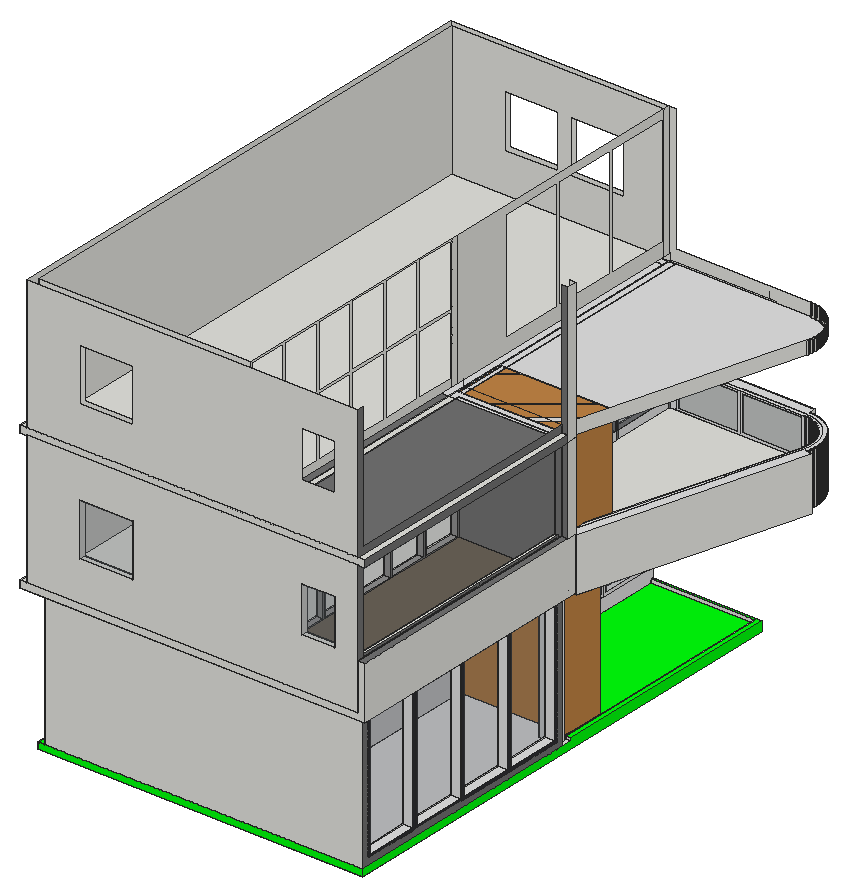
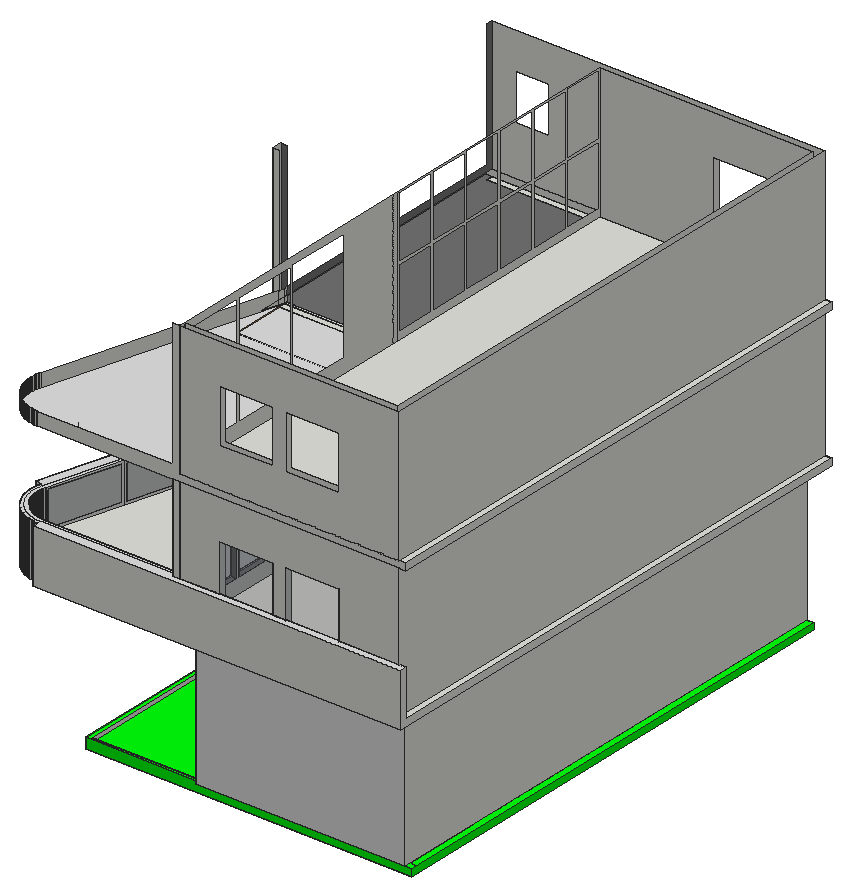
# SketchUp Ruby script. Lengths in inches.
U = 1.inch
M = Sketchup.active_model
def pt(a) = Geom::Point3d.new(a.map { |v| v * U })
def face(e, loops, mat)
  f = e.add_face(loops[0].map { |a| pt(a) })
  loops[1..].each { |l| e.add_face(l.map { |a| pt(a) }).erase! }
  f.material = f.back_material = mat if mat
  f
end
# faces: each face lists its corners as indices into pts; further lists are holes
def faces(e, pts, list, mat = nil) = list.each { |f| face(e, (f[0].is_a?(Array) ? f : [f]).map { |l| l.map { |i| pts[i] } }, mat) }
# xy, xz, yz: faces in a plane at the given z, y or x. An outline is a flat list of corners, or four numbers for a rectangle; further outlines are holes
def ring(l) = l.size == 4 ? [[l[0], l[1]], [l[2], l[1]], [l[2], l[3]], [l[0], l[3]]] : l.each_slice(2).to_a
def flat(e, list, mat, &to3) = list.each { |f| face(e, (f[0].is_a?(Array) ? f : [f]).map { |l| ring(l).map { |u, v| to3.(u, v) } }, mat) }
def xy(e, z, list, mat = nil) = flat(e, list, mat) { |x, y| [x, y, z] }
def xz(e, y, list, mat = nil) = flat(e, list, mat) { |x, z| [x, y, z] }
def yz(e, x, list, mat = nil) = flat(e, list, mat) { |y, z| [x, y, z] }
def lines(e, pts, list) = list.each { |a, b| e.add_line(pt(pts[a]), pt(pts[b])) }
# prism: a flat outline (further loops are holes) pulled along v
def prism(e, loops, v, mat = nil)
  f = face(e, loops, mat); d = Geom::Vector3d.new(v.map { |x| x * U })
  f.pushpull(f.normal.samedirection?(d) ? d.length : -d.length)
end
def box(e, o, s, mat = nil) = prism(e, [[o, [o[0] + s[0], o[1], o[2]], [o[0] + s[0], o[1] + s[1], o[2]], [o[0], o[1] + s[1], o[2]]]], [0, 0, s[2]], mat)
def at(x, y, z, deg = 0) = Geom::Transformation.translation(pt([x, y, z])) * Geom::Transformation.rotation(ORIGIN, Z_AXIS, deg.degrees)
def axes(o, x, y, z) = Geom::Transformation.new([*x, 0, *y, 0, *z, 0, *pt(o).to_a, 1])
def part(name) = M.definitions.add(name)
# library, detail: a bought-in or finely detailed component or shape, given as its bounding box
def library(name, o, s) = part(name).tap { |d| box(d.entities, o, s) }
def detail(e, o, s) = box(e.add_group.entities, o, s)
def put(e, d, t, mat = nil) = e.add_instance(d, t).tap { |i| i.material = mat if mat }
def group(e, t, mat = nil) = e.add_group.tap { |g| g.transformation = t; g.material = mat if mat }.entities
root = M.entities
M.materials.add("Glass_Basic_01").color = [105, 113, 122]
M.materials["Glass_Basic_01"].alpha = 0.25
M.materials.add("M01_Silver_Fog").color = [224, 224, 224]
M.materials.add("M04_Stone_Frost").color = [142, 142, 142]
M.materials.add("M06_Steel_Smoke").color = [114, 114, 114]
M.materials.add("Plaster_04_1K").color = [106, 98, 87]
M.materials.add("Roofing_02_1K").color = [0, 255, 11]
M.materials.add("ThomThom - Buttons1").color = [48, 49, 53]
M.materials.add("Wood_Floor_01_1K").color = [193, 132, 69]
c1 = part("Group\#1")
box(c1.entities,[-3.94,0,0],[99.94,48,114])
xy(root,0,[[9,9,303,462]])
xy(root,6,[[15,9,24,456],[24,9,303,18],[198,18,204,213],[204,18,303,213],[297,235.29,303,235.29,303,245.13,294,245.13,294,244.03,299.12,242.53],
  [204,244.03,294,245.13],[15,456,204,462]])
xy(root,6,[[24,18,198,456],[198,213,204,245.13],[204,213,204,244.03,294,244.03,299.12,242.53,297,235.29,303,235.29,303,213],[198,245.13,204,456]],"M01_Silver_Fog")
xy(root,6,[[9,9,15,456],[204,245.13,298.5,459.53],[9,456,15,462]],"Roofing_02_1K")
xy(root,9,[[298.5,245.13,303,245.13,303,462,204,462,204,459.53,298.5,459.53]],"Roofing_02_1K")
xy(root,12,[[204,18,294,18,294,227.29,288,227.29,288,236.58,290.18,244.03,204,244.03],[288,227.29,288,236.58,290.18,244.03,294,244.03,294,227.29],[290.18,244.03,290.48,245.06,294,244.03]],"M01_Silver_Fog")
xy(root,14,[[294,17,303,66.57],[294,70.57,303,120.15],[294,124.15,303,173.72],[294,177.72,303,227.29]],"M01_Silver_Fog")
xy(root,20,[[198,308.82,204,354.55],[198,358.55,204,404.27],[198,408.27,204,454]],"M01_Silver_Fog")
xy(root,124,[[294,17,303,66.57],[294,70.57,303,120.15],[294,124.15,303,173.72],[294,177.72,303,227.29],[198,308.82,204,354.55],
  [198,358.55,204,404.27],[198,408.27,204,454]],"M01_Silver_Fog")
xy(root,132,[[306,231,306,234,307.76,240,312,238.76,312,231],[312,238.76,307.76,240,312,240]])
xy(root,132,[[[0,0,0,486,331.55,486,331.55,480,332.69,479.96,334.03,479.87,335.37,479.72,336.7,479.52,338.02,479.28,339.33,478.98,340.63,478.63,341.92,478.23,343.1875,477.79,344.44,477.29,345.67,476.75,346.88,476.16,348.07,475.53,349.23,474.85,350.37,474.13,351.47,473.37,352.55,472.5625,353.6,471.72,354.61,470.83,355.59,469.91,356.53,468.95,357.39,468,357.4375,467.95,358.3,466.92,359.13,465.86,359.92,464.77,360.66,463.65,360.69,463.59,361.36,462.5,362.02,461.33,362.63,460.13,363.2,458.91,363.71,457.67,364.18,456.41,364.61,455.13,364.98,453.84,365.3,452.53,365.58,451.21,365.8,449.89,365.98,448.55,366.1,447.21,366.17,445.87,366.1875,444.52,366.16,443.18,366.07,441.84,365.94,440.5,365.76,439.16,365.52,437.84,365.24,436.52,364.95,435.42,370.71,433.74,313.51,238.31,312,238.76,312,240,307.76,240,306,234,306,231,312,231,312,0],[15,9,303,9,303,235.29,297,235.29,299.12,242.53,290.48,245.06,347.59,440.19,347.64,440.34,347.63,440.34,347.72,440.68,347.86,441.32,347.97,441.97,348.0625,442.625,348.13,443.28,348.17,443.94,348.19,444.6,348.18,445.26,348.14,445.92,348.08,446.58,348,447.23,347.89,447.88,347.75,448.53,347.59,449.17,347.41,449.8,347.2,450.43,346.97,451.05,346.72,451.66,346.44,452.25,346.14,452.84,345.82,453.42,345.47,453.98,345.11,454.53,344.72,455.07,344.32,455.59,343.89,456.09,343.45,456.58,342.99,457.05,342.51,457.5,342.01,457.9375,341.5,458.35,340.97,458.75,340.42,459.125,339.87,459.48,339.3,459.81,338.72,460.12,338.12,460.41,337.52,460.67,336.9,460.92,336.28,461.13,335.65,461.33,335.01,461.5,334.37,461.65,333.72,461.77,333.07,461.86,332.41,461.9375,331.75,461.98,331.25,462,15,462]],[24,18,198,456],[204,18,204,462,331.25,462,331.75,461.98,332.41,461.9375,333.07,461.86,333.72,461.77,334.37,461.65,335.01,461.5,335.65,461.33,336.28,461.13,336.9,460.92,337.52,460.67,338.12,460.41,338.72,460.12,339.3,459.81,339.87,459.48,340.42,459.125,340.97,458.75,341.5,458.35,342.01,457.9375,342.51,457.5,342.99,457.05,343.45,456.58,343.89,456.09,344.32,455.59,344.72,455.07,345.11,454.53,345.47,453.98,345.82,453.42,346.14,452.84,346.44,452.25,346.72,451.66,346.97,451.05,347.2,450.43,347.41,449.8,347.59,449.17,347.75,448.53,347.89,447.88,348,447.23,348.08,446.58,348.14,445.92,348.18,445.26,348.19,444.6,348.17,443.94,348.13,443.28,348.0625,442.625,347.97,441.97,347.86,441.32,347.72,440.68,347.63,440.34,347.59,440.19,290.48,245.06,288,236.58,288,227.29,294,227.29,294,18]],"M01_Silver_Fog")
xy(root,138,[[0,0,6,480],[12,6,204,474]])
xy(root,144,[[303,6,306,231],[306,234,307.76,240,306,240],[216,246,303.26,246,306,255.36,321.22,307.35,340.07,371.78,359.17,437.01,359.4,437.91,359.63,439,359.83,440.1,359.98,441.21,360.09,442.32,360.16,443.43,360.1875,444.55,360.17,445.67,360.11,446.78,360.01,447.89,359.87,449,359.68,450.1,359.45,451.2,359.18,452.28,358.875,453.35,358.52,454.41,358.13,455.46,357.7,456.49,357.23,457.5,356.73,458.5,356.18,459.47,355.6,460.43,354.98,461.36,354.33,462.26,353.64,463.14,352.92,464,352.17,464.83,351.39,465.62,350.58,466.39,349.74,467.125,348.87,467.83,347.97,468.5,347.05,469.13,346.11,469.73,345.15,470.29,344.16,470.82,343.16,471.3,342.13,471.75,341.09,472.16,340.04,472.53,338.97,472.86,337.89,473.15,336.8,473.4,335.71,473.6,334.6,473.77,333.49,473.89,332.38,473.97,331.45,474,210,474,210,288,213,288,213,287.79,216,287.79]])
xy(root,144,[[210,6,300,234]],"Plaster_04_1K")
xy(root,145,[[204,7,210,43],[204,45,210,81],[204,83,210,119],[204,121,210,157],[204,159,210,195],
  [204,197,210,233]],"M04_Stone_Frost")
xy(root,146,[[300,8,303,49],[300,53,303,94],[300,98,303,139],[300,143,303,184],[300,188,303,229]])
xy(root,151,[[204,295,210,353],[204,355,210,413],[204,415,210,473]],"M06_Steel_Smoke")
xy(root,174,[[54,0,102,6],[60,474,108,480],[120,474,168,480]])
xy(root,178,[[300,8,303,49],[300,53,303,94],[300,98,303,139],[300,143,303,184],[300,188,303,229]])
xy(root,180,[[300,6,303,231]])
xy(root,180,[[313.51,238.31,370.71,433.74,364.95,435.42,362.06,436.22,361.5,434.3,343.76,373.7,342.64,369.86,324.9,309.27,323.78,305.43,306.07,244.92,305.51,243,213,243,213,288,210,288,210,240,312,240,312,238.76],[312,238.76,312,240,307.76,240],[213,243,305.51,243,306.07,244.92,323.78,305.43,324.9,309.27,342.64,369.86,343.2,371.78,340.07,371.78,321.22,307.35,306,255.36,303.26,246,216,246,216,287.79,213,287.79],[340.07,371.78,343.2,371.78,343.76,373.7,361.5,434.3,362.06,436.22,362.32,437.22,362.58,438.42,362.79,439.63,362.96,440.85,363.08,442.08,363.16,443.31,363.1875,444.54,363.17,445.77,363.1,447,362.99,448.22,362.83,449.44,362.63,450.66,362.38,451.86,362.08,453.06,361.74,454.24,361.35,455.41,360.92,456.5625,360.45,457.7,359.93,458.82,359.37,459.91,358.77,460.99,358.13,462.03,358.13,462.04,357.45,463.0625,356.73,464.0625,355.97,465.03,355.18,465.98,355.17,465.98,354.35,466.89,353.49,467.76,352.59,468.61,351.67,469.42,350.71,470.19,349.72,470.93,348.71,471.63,347.67,472.29,346.61,472.91,345.52,473.49,344.41,474.03,343.29,474.52,342.14,474.97,340.98,475.38,339.8,475.75,338.61,476.0625,337.41,476.34,336.2,476.5625,334.99,476.74,333.76,476.88,332.53,476.97,331.5,477,210,477,210,474,331.45,474,332.38,473.97,333.49,473.89,334.6,473.77,335.71,473.6,336.8,473.4,337.89,473.15,338.97,472.86,340.04,472.53,341.09,472.16,342.13,471.75,343.16,471.3,344.16,470.82,345.15,470.29,346.11,469.73,347.05,469.13,347.97,468.5,348.87,467.83,349.74,467.125,350.58,466.39,351.39,465.62,352.17,464.83,352.92,464,353.64,463.14,354.33,462.26,354.98,461.36,355.6,460.43,356.18,459.47,356.73,458.5,357.23,457.5,357.7,456.49,358.13,455.46,358.52,454.41,358.875,453.35,359.18,452.28,359.45,451.2,359.68,450.1,359.87,449,360.01,447.89,360.11,446.78,360.17,445.67,360.1875,444.55,360.16,443.43,360.09,442.32,359.98,441.21,359.83,440.1,359.63,439,359.4,437.91,359.17,437.01],[364.95,435.42,365.24,436.52,365.52,437.84,365.76,439.16,365.94,440.5,366.07,441.84,366.16,443.18,366.1875,444.52,366.17,445.87,366.1,447.21,365.98,448.55,365.8,449.89,365.58,451.21,365.3,452.53,364.98,453.84,364.61,455.13,364.18,456.41,363.71,457.67,363.2,458.91,362.63,460.13,362.02,461.33,361.36,462.5,360.69,463.59,360.66,463.65,359.92,464.77,359.13,465.86,358.3,466.92,357.4375,467.95,357.39,468,356.53,468.95,355.59,469.91,354.61,470.83,353.6,471.72,352.55,472.5625,351.47,473.37,350.37,474.13,349.23,474.85,348.07,475.53,346.88,476.16,345.67,476.75,344.44,477.29,343.1875,477.79,341.92,478.23,340.63,478.63,339.33,478.98,338.02,479.28,336.7,479.52,335.37,479.72,334.03,479.87,332.69,479.96,331.55,480,331.55,486,0,486,0,480,210,480,210,477,331.5,477,332.53,476.97,333.76,476.88,334.99,476.74,336.2,476.5625,337.41,476.34,338.61,476.0625,339.8,475.75,340.98,475.38,342.14,474.97,343.29,474.52,344.41,474.03,345.52,473.49,346.61,472.91,347.67,472.29,348.71,471.63,349.72,470.93,350.71,470.19,351.67,469.42,352.59,468.61,353.49,467.76,354.35,466.89,355.17,465.98,355.18,465.98,355.97,465.03,356.73,464.0625,357.45,463.0625,358.13,462.04,358.13,462.03,358.77,460.99,359.37,459.91,359.93,458.82,360.45,457.7,360.92,456.5625,361.35,455.41,361.74,454.24,362.08,453.06,362.38,451.86,362.63,450.66,362.83,449.44,362.99,448.22,363.1,447,363.17,445.77,363.1875,444.54,363.16,443.31,363.08,442.08,362.96,440.85,362.79,439.63,362.58,438.42,362.32,437.22,362.06,436.22]],"M01_Silver_Fog")
xy(root,180,[[306,0,312,231]],"M06_Steel_Smoke")
xy(root,183,[[255,0,285,6]])
xy(root,199,[[204,7,210,43],[204,45,210,81],[204,83,210,119],[204,121,210,157],[204,159,210,195],
  [204,197,210,233]])
xy(root,201,[[204,7,210,43],[204,45,210,81],[204,83,210,119],[204,121,210,157],[204,159,210,195],
  [204,197,210,233]],"M04_Stone_Frost")
xy(root,222,[[54,0,102,6],[60,474,108,480],[120,474,168,480]])
xy(root,225,[[255,0,285,6]])
xy(root,251,[[204,295,210,353],[204,355,210,413],[204,415,210,473]],"M06_Steel_Smoke")
xy(root,257,[[204,7,210,43],[204,45,210,81],[204,83,210,119],[204,121,210,157],[204,159,210,195],
  [204,197,210,233]])
xy(root,258,[[0,0,6,231],[6,0,306,0,306,6,210,6,210,234,306,234,306,240,210,240,210,480,204,480,204,6,12,6,12,474,204,474,204,480,6,480],[0,231,6,480],[300,231,306,234],[306,231,306,234,307.76,240,312,240,312,231]])
xy(root,258,[[6,231,6,480,210,480,210,240,306,240,306,234,210,234,210,231,204,231,204,474,12,474,12,231],[12,231,204,474],[210,231,300,234],[306,234,306,240,210,240,210,480,331.55,480,332.69,479.96,334.03,479.87,335.37,479.72,336.7,479.52,338.02,479.28,339.33,478.98,340.63,478.63,341.92,478.23,343.1875,477.79,344.44,477.29,345.67,476.75,346.88,476.16,348.07,475.53,349.23,474.85,350.37,474.13,351.47,473.37,352.55,472.5625,353.6,471.72,354.61,470.83,355.59,469.91,356.53,468.95,357.39,468,357.4375,467.95,358.3,466.92,359.13,465.86,359.92,464.77,360.66,463.65,360.69,463.59,361.36,462.5,362.02,461.33,362.63,460.13,363.2,458.91,363.71,457.67,364.18,456.41,364.61,455.13,364.98,453.84,365.3,452.53,365.58,451.21,365.8,449.89,365.98,448.55,366.1,447.21,366.17,445.87,366.1875,444.52,366.16,443.18,366.07,441.84,365.94,440.5,365.76,439.16,365.52,437.84,365.24,436.52,364.95,435.42,307.76,240]],"M01_Silver_Fog")
xy(root,258,[[6,0,6,231,12,231,12,6,204,6,204,231,210,231,210,6,306,6,306,0],[306,0,306,6,210,6,210,231,312,231,312,0],[12,6,204,231]],"M06_Steel_Smoke")
xy(root,258.01,[[306,231,312,240]])
xy(root,264,[[0,0,6,480],[306,0,312,231],[12,6,204,474]])
xz(root,0,[[0,132,312,132,312,180,306,180,306,138,0,138],[[6,138,306,258],[54,174,102,222],[255,183,285,225]],[0,258,312,264],[[6,264,306,384],[54,300,102,348],[255,309,285,351]]])
xz(root,0,[[54,174,102,222],[255,183,285,225]],"Glass_Basic_01")
xz(root,6,[[[12,138,204,258],[54,174,102,222]],[[252,180,288,228],[255,183,285,225]],[[12,264,204,384],[54,300,102,348]]])
xz(root,6,[[[210,144,210,258,306,258,306,144,303,144,303,180,300,180,300,144],[252,180,288,228]]],"M06_Steel_Smoke")
xz(root,7,[[204,145,210,199],[204,201,210,257]],"M04_Stone_Frost")
xz(root,8,[[300,146,303,178]])
xz(root,9,[[15,6,303,132]])
xz(root,9,[[9,0,303,6]],"Roofing_02_1K")
xz(root,17,[[294,14,303,124]],"M01_Silver_Fog")
xz(root,18,[[24,6,198,12]])
xz(root,18,[[198,6,204,12],[24,12,198,132],[204,12,294,132]],"M01_Silver_Fog")
xz(root,43,[[204,145,210,199],[204,201,210,257]],"M04_Stone_Frost")
xz(root,45,[[204,145,210,199],[204,201,210,257]],"M04_Stone_Frost")
xz(root,49,[[300,146,303,178]])
xz(root,53,[[300,146,303,178]])
xz(root,66.57,[[294,14,303,124]],"M01_Silver_Fog")
xz(root,70.57,[[294,14,303,124]],"M01_Silver_Fog")
xz(root,81,[[204,145,210,199],[204,201,210,257]],"M04_Stone_Frost")
xz(root,83,[[204,145,210,199],[204,201,210,257]],"M04_Stone_Frost")
xz(root,94,[[300,146,303,178]])
xz(root,98,[[300,146,303,178]])
xz(root,119,[[204,145,210,199],[204,201,210,257]],"M04_Stone_Frost")
xz(root,120.15,[[294,14,303,124]],"M01_Silver_Fog")
xz(root,121,[[204,145,210,199],[204,201,210,257]],"M04_Stone_Frost")
xz(root,124.15,[[294,14,303,124]],"M01_Silver_Fog")
xz(root,139,[[300,146,303,178]])
xz(root,143,[[300,146,303,178]])
xz(root,157,[[204,145,210,199],[204,201,210,257]],"M04_Stone_Frost")
xz(root,159,[[204,145,210,199],[204,201,210,257]],"M04_Stone_Frost")
xz(root,173.72,[[294,14,303,124]],"M01_Silver_Fog")
xz(root,177.72,[[294,14,303,124]],"M01_Silver_Fog")
xz(root,184,[[300,146,303,178]])
xz(root,188,[[300,146,303,178]])
xz(root,195,[[204,145,210,199],[204,201,210,257]],"M04_Stone_Frost")
xz(root,197,[[204,145,210,199],[204,201,210,257]],"M04_Stone_Frost")
xz(root,227.29,[[288,12,294,132],[294,14,303,124]],"M01_Silver_Fog")
xz(root,229,[[300,146,303,178]])
xz(root,231,[[306,258.01,312,264]])
xz(root,231,[[303,144,306,144,306,258,300,258,300,180,303,180],[306,180,312,258],[306,258,312,258.01],[306,264,312,384]],"M06_Steel_Smoke")
xz(root,233,[[204,145,210,199],[204,201,210,257]],"M04_Stone_Frost")
xz(root,234,[[300,144,306,258]])
xz(root,234,[[210,144,300,258]],"M06_Steel_Smoke")
xz(root,235.29,[[297,6,303,132]],"M01_Silver_Fog")
xz(root,240,[[307.76,132,312,180],[306,180,306,258.01,307.76,258.01,307.76,258,312,258,312,180],[307.76,258,312,258.01],[307.76,258.01,307.76,270,306,270,306,384.01,307.76,384.01,307.76,384,312,384,312,258.01]])
xz(root,240,[[210,144,306,180],[306,144,307.76,180]],"M01_Silver_Fog")
xz(root,244.03,[[204,6,294,12]],"M01_Silver_Fog")
xz(root,245.13,[[298.5,6,303,9]])
xz(root,246,[[216,144,303.26,180]],"M01_Silver_Fog")
xz(root,287.79,[[213,144,216,180]],"M01_Silver_Fog")
xz(root,288,[[210,144,213,180]],"M01_Silver_Fog")
xz(root,295,[[204,151,210,251]],"M06_Steel_Smoke")
xz(root,308.82,[[198,20,204,124]],"M01_Silver_Fog")
xz(root,353,[[204,151,210,251]],"M06_Steel_Smoke")
xz(root,354.55,[[198,20,204,124]],"M01_Silver_Fog")
xz(root,355,[[204,151,210,251]],"M06_Steel_Smoke")
xz(root,358.55,[[198,20,204,124]],"M01_Silver_Fog")
xz(root,404.27,[[198,20,204,124]],"M01_Silver_Fog")
xz(root,408.27,[[198,20,204,124]],"M01_Silver_Fog")
xz(root,413,[[204,151,210,251]],"M06_Steel_Smoke")
xz(root,415,[[204,151,210,251]],"M06_Steel_Smoke")
xz(root,454,[[198,20,204,124]],"M01_Silver_Fog")
xz(root,456,[[24,6,198,132]],"M01_Silver_Fog")
xz(root,459.53,[[204,6,298.5,9]])
xz(root,462,[[15,6,204,132]],"M01_Silver_Fog")
xz(root,462,[[9,0,9,6,204,6,204,9,303,9,303,0]],"Roofing_02_1K")
xz(root,473,[[204,151,210,251]],"M06_Steel_Smoke")
xz(root,474,[[[12,138,204,258],[120,174,168,222],[60,174,108,222]],[[12,264,204,384],[120,300,168,348],[60,300,108,348]]])
xz(root,474,[[218,146,271.49,178],[275.49,146,329.45,178]],"Glass_Basic_01")
xz(root,474,[[210,144,215.53,180],[215.53,144,216,180],[[216,144,273.49,180],[218,146,271.49,178]],[[273.49,144,331.45,180],[275.49,146,329.45,178]]],"M01_Silver_Fog")
xz(root,477,[[274.25,178,329.5,180]],"Glass_Basic_01")
xz(root,480,[[0,138,6,180],[6,138,204,138,204,180,168,180,168,174,120,174,120,180,108,180,108,174,60,174,60,180,6,180],[6,180,6,258,204,258,204,180,168,180,168,222,120,222,120,180,108,180,108,222,60,222,60,180],[204,180,210,258],[0,258,0,264,204,264,204,384,210,384,210,270,331.55,270,331.55,258],
  [[6,264,204,384],[60,300,108,348],[120,300,168,348]]])
xz(root,480,[[60,174,108,180],[120,174,168,180],[60,180,108,222],[120,180,168,222]],"Glass_Basic_01")
xz(root,486,[[0,132,331.55,180]])
yz(root,0,[[0,132,0,138,480,138,480,180,486,180,486,132],[0,258,480,264]])
yz(root,6,[[0,138,480,258],[0,264,480,384]])
yz(root,9,[[9,0,462,6]],"Roofing_02_1K")
yz(root,12,[[6,138,474,258],[6,264,474,384]])
yz(root,15,[[9,6,462,132]])
yz(root,24,[[18,6,456,132]],"M01_Silver_Fog")
yz(root,54,[[0,174,6,222]])
yz(root,60,[[474,174,480,222]])
yz(root,102,[[0,174,6,222]])
yz(root,108,[[474,174,480,222]])
yz(root,120,[[474,174,480,222]])
yz(root,168,[[474,174,480,222]])
yz(root,198,[[[18,6,456,132],[358.55,20,404.27,124],[308.82,20,354.55,124],[408.27,20,454,124]]],"M01_Silver_Fog")
yz(root,204,[[459.53,6,462,9],[[6,138,234,258],[7,201,43,257],[121,201,157,257],[159,201,195,257],[197,201,233,257],[45,201,81,257],[83,201,119,257],[7,145,43,199],[197,145,233,199],[159,145,195,199],[121,145,157,199],[45,145,81,199],[83,145,119,199]],[234,138,240,258],[[240,138,474,258],[415,151,473,251],[295,151,353,251],[355,151,413,251]],[474,138,480,258],
  [[6,264,234,384],[7,327,43,383],[121,327,157,383],[159,327,195,383],[197,327,233,383],[45,327,81,383],[83,327,119,383],[7,271,43,325],[197,271,233,325],[159,271,195,325],[121,271,157,325],[45,271,81,325],[83,271,119,325]],[234,264,240,384],[[240,264,474,384],[415,277,473,377],[295,277,353,377],[355,277,413,377]],[474,264,480,384]])
yz(root,204,[[308.82,20,354.55,124],[358.55,20,404.27,124],[408.27,20,454,124],[7,145,43,199],[45,145,81,199],
  [83,145,119,199],[121,145,157,199],[159,145,195,199],[197,145,233,199],[295,151,353,251],
  [355,151,413,251],[415,151,473,251],[7,201,43,257],[45,201,81,257],[83,201,119,257],
  [121,201,157,257],[159,201,195,257],[197,201,233,257]],"Glass_Basic_01")
yz(root,204,[[18,6,244.03,12],[[244.03,6,459.53,6,459.53,9,462,9,462,132,18,132,18,12,244.03,12],[306.82,18,456,126]],[[306.82,18,356.55,126],[308.82,20,354.55,124]],[[356.55,18,406.27,126],[358.55,20,404.27,124]],[[406.27,18,456,126],[408.27,20,454,124]]],"M01_Silver_Fog")
yz(root,210,[[240,180,288,180,288,190.46,286.46,190.46,286.46,211.54,288,211.54,288,258,240,258],[286.46,190.46,288,211.54]])
yz(root,210,[[295,151,353,251],[355,151,413,251],[415,151,473,251]],"Glass_Basic_01")
yz(root,210,[[295,144,353,151],[355,144,413,151],[415,144,473,151]],"M01_Silver_Fog")
yz(root,210,[[6,144,44,144,44,201,43,201,43,145,7,145,7,257,43,257,43,201,44,201,44,258,6,258],[44,144,82,144,82,201,81,201,81,145,45,145,45,201,44,201],[82,144,120,144,120,201,119,201,119,145,83,145,83,201,82,201],[120,144,158,144,158,201,157,201,157,145,121,145,121,201,120,201],[158,144,196,144,196,201,195,201,195,145,159,145,159,201,158,201],
  [196,144,234,144,234,258,196,258,196,201,197,201,197,257,233,257,233,145,197,145,197,201,196,201],[288,144,294,144,294,252,474,252,474,180,480,180,480,258,288,258],[294,144,295,144,295,251,353,251,353,144,354,144,354,252,294,252],[354,144,355,144,355,251,413,251,413,144,414,144,414,252,354,252],[414,144,415,144,415,251,473,251,473,144,474,144,474,252,414,252],
  [474,144,477,180],[7,199,43,201],[45,199,81,201],[83,199,119,201],[121,199,157,201],
  [159,199,195,201],[197,199,233,201],[44,201,45,201,45,257,81,257,81,201,82,201,82,258,44,258],[82,201,83,201,83,257,119,257,119,201,120,201,120,258,82,258],[120,201,121,201,121,257,157,257,157,201,158,201,158,258,120,258],
  [158,201,159,201,159,257,195,257,195,201,196,201,196,258,158,258]],"M06_Steel_Smoke")
yz(root,213,[[287.79,144,288,180]],"M01_Silver_Fog")
yz(root,216,[[246,144,287.79,180]],"M01_Silver_Fog")
yz(root,255,[[0,183,6,225]])
yz(root,285,[[0,183,6,225]])
yz(root,288,[[227.29,12,236.58,132]],"M01_Silver_Fog")
yz(root,294,[[18,14,66.57,124],[70.57,14,120.15,124],[124.15,14,173.72,124],[177.72,14,227.29,124]],"Glass_Basic_01")
yz(root,294,[[[18,12,18,14,66.57,14,66.57,124,18,124,18,132,227.29,132,227.29,124,124.15,124,124.15,14,227.29,14,227.29,12],[70.57,14,120.15,124]],[17,14,18,124],[173.72,14,177.72,124]],"M01_Silver_Fog")
yz(root,298.5,[[245.13,6,459.53,9]])
yz(root,300,[[[6,144,231,180],[8,146,49,178],[143,146,184,178],[188,146,229,178],[53,146,94,178],[98,146,139,178]],[231,144,234,258]])
yz(root,300,[[8,146,49,178],[53,146,94,178],[98,146,139,178],[143,146,184,178],[188,146,229,178]],"Glass_Basic_01")
yz(root,303,[[8,146,49,178],[53,146,94,178],[98,146,139,178],[143,146,184,178],[188,146,229,178]],"Glass_Basic_01")
yz(root,303,[[[9,6,235.29,132],[15,12,229.29,126]],[[6,144,51,180],[8,146,49,178]],[[51,144,96,180],[53,146,94,178]],[[96,144,141,180],[98,146,139,178]],[[141,144,186,180],[143,146,184,178]],
  [[186,144,231,180],[188,146,229,178]]],"M06_Steel_Smoke")
yz(root,303,[[9,0,462,0,462,9,245.13,9,245.13,6,9,6]],"Roofing_02_1K")
yz(root,303,[[[15,12,68.57,126],[17,14,66.57,124]],[[68.57,12,122.15,126],[70.57,14,120.15,124]],[[122.15,12,175.72,126],[124.15,14,173.72,124]],[[175.72,12,229.29,126],[177.72,14,227.29,124]]],"ThomThom - Buttons1")
yz(root,306,[[231,132,234,138],[0,138,234,144],[231,144,234,258],[231,258,234,258.01],[234,258,240,258.01],
  [231,258.01,234,264],[231,264,234,270]])
yz(root,306,[[0,144,6,180],[6,144,231,180],[0,180,6,258],[0,264,231,264,231,270,6,270,6,384,0,384]],"M06_Steel_Smoke")
yz(root,312,[[0,132,240,180],[231,180,240,258],[231,258,240,258.01],[231,258.01,240,384]])
yz(root,312,[[0,258,231,264]],"M06_Steel_Smoke")
yz(root,331.55,[[480,132,486,180]])
p = [[299.12,242.53,132],[297,235.29,132],[297,235.29,6],[299.12,242.53,6],[294,244.03,6],[294,244.03,12],
  [290.48,245.06,12],[290.48,245.06,132],[288,236.58,132],[290.18,244.03,12],[288,236.58,12],[306,234,132],
  [307.76,240,132],[307.76,240,144],[306,234,144],[306,234,138],[307.76,240,180],[312,238.76,132],
  [313.51,238.31,132],[313.51,238.31,180],[312,238.76,180],[370.71,433.74,132],[370.71,433.74,180],[364.95,435.42,132],
  [364.95,435.42,180],[365.24,436.52,132],[365.24,436.52,180],[365.52,437.84,132],[365.52,437.84,180],[365.76,439.16,132],
  [365.76,439.16,180],[365.94,440.5,132],[365.94,440.5,180],[366.07,441.84,132],[366.07,441.84,180],[366.16,443.18,132],
  [366.16,443.18,180],[366.1875,444.52,132],[366.1875,444.52,180],[366.17,445.87,132],[366.17,445.87,180],[366.1,447.21,132],
  [366.1,447.21,180],[365.98,448.55,132],[365.98,448.55,180],[365.8,449.89,132],[365.8,449.89,180],[365.58,451.21,132],
  [365.58,451.21,180],[365.3,452.53,132],[365.3,452.53,180],[364.98,453.84,132],[364.98,453.84,180],[364.61,455.13,132],
  [364.61,455.13,180],[364.18,456.41,132],[364.18,456.41,180],[363.71,457.67,132],[363.71,457.67,180],[363.2,458.91,132],
  [363.2,458.91,180],[362.63,460.13,132],[362.63,460.13,180],[362.02,461.33,132],[362.02,461.33,180],[361.36,462.5,132],
  [361.36,462.5,180],[360.69,463.59,132],[360.69,463.59,180],[359.92,464.77,132],[359.92,464.77,180],[360.66,463.65,180],
  [360.66,463.65,132],[359.13,465.86,132],[359.13,465.86,180],[358.3,466.92,132],[358.3,466.92,180],[357.4375,467.95,132],
  [357.4375,467.95,180],[356.53,468.95,132],[356.53,468.95,180],[357.39,468,180],[357.39,468,132],[355.59,469.91,132],
  [355.59,469.91,180],[354.61,470.83,132],[354.61,470.83,180],[353.6,471.72,132],[353.6,471.72,180],[352.55,472.5625,132],
  [352.55,472.5625,180],[351.47,473.37,132],[351.47,473.37,180],[350.37,474.13,132],[350.37,474.13,180],[349.23,474.85,132],
  [349.23,474.85,180],[348.07,475.53,132],[348.07,475.53,180],[346.88,476.16,132],[346.88,476.16,180],[345.67,476.75,132],
  [345.67,476.75,180],[344.44,477.29,132],[344.44,477.29,180],[343.1875,477.79,132],[343.1875,477.79,180],[341.92,478.23,132],
  [341.92,478.23,180],[340.63,478.63,132],[340.63,478.63,180],[339.33,478.98,132],[339.33,478.98,180],[338.02,479.28,132],
  [338.02,479.28,180],[336.7,479.52,132],[336.7,479.52,180],[335.37,479.72,132],[335.37,479.72,180],[334.03,479.87,132],
  [334.03,479.87,180],[332.69,479.96,132],[332.69,479.96,180],[331.55,480,132],[331.55,480,180],[303.26,246,180],
  [306,255.36,180],[306,255.36,144],[303.26,246,144],[321.22,307.35,180],[321.22,307.35,144],[320.65,305.43,178],
  [306.5625,257.28,178],[306.5625,257.28,146],[320.65,305.43,146],[340.07,371.78,180],[340.07,371.78,144],[339.51,369.86,146],
  [339.51,369.86,178],[321.78,309.27,178],[321.78,309.27,146],[359.17,437.01,144],[359.17,437.01,180],[340.64,373.7,146],
  [358.6,435.09,146],[358.6,435.09,178],[340.64,373.7,178],[359.4,437.91,144],[359.4,437.91,180],[359.63,439,144],
  [359.63,439,180],[359.83,440.1,144],[359.83,440.1,180],[359.98,441.21,144],[359.98,441.21,180],[360.09,442.32,144],
  [360.09,442.32,180],[360.16,443.43,144],[360.16,443.43,180],[360.1875,444.55,144],[360.1875,444.55,180],[360.17,445.67,144],
  [360.17,445.67,180],[360.11,446.78,144],[360.11,446.78,180],[360.01,447.89,144],[360.01,447.89,180],[359.87,449,144],
  [359.87,449,180],[359.68,450.1,144],[359.68,450.1,180],[359.45,451.2,144],[359.45,451.2,180],[359.18,452.28,144],
  [359.18,452.28,180],[358.875,453.35,144],[358.875,453.35,180],[358.52,454.41,144],[358.52,454.41,180],[358.13,455.46,144],
  [358.13,455.46,180],[357.7,456.49,144],[357.7,456.49,180],[357.23,457.5,144],[357.23,457.5,180],[356.73,458.5,144],
  [356.73,458.5,180],[356.18,459.47,144],[356.18,459.47,180],[355.6,460.43,144],[355.6,460.43,180],[354.98,461.36,144],
  [354.98,461.36,180],[354.33,462.26,144],[354.33,462.26,180],[353.64,463.14,144],[353.64,463.14,180],[352.92,464,144],
  [352.92,464,180],[352.17,464.83,144],[352.17,464.83,180],[351.39,465.62,144],[351.39,465.62,180],[350.58,466.39,144],
  [350.58,466.39,180],[349.74,467.125,144],[349.74,467.125,180],[348.87,467.83,144],[348.87,467.83,180],[347.97,468.5,144],
  [347.97,468.5,180],[347.05,469.13,144],[347.05,469.13,180],[346.11,469.73,144],[346.11,469.73,180],[345.15,470.29,144],
  [345.15,470.29,180],[344.16,470.82,144],[344.16,470.82,180],[343.16,471.3,144],[343.16,471.3,180],[342.13,471.75,144],
  [342.13,471.75,180],[341.09,472.16,144],[341.09,472.16,180],[340.04,472.53,144],[340.04,472.53,180],[338.97,472.86,144],
  [338.97,472.86,180],[337.89,473.15,144],[337.89,473.15,180],[336.8,473.4,144],[336.8,473.4,180],[335.71,473.6,144],
  [335.71,473.6,180],[334.6,473.77,144],[334.6,473.77,180],[333.49,473.89,144],[333.49,473.89,180],[332.38,473.97,144],
  [332.38,473.97,180],[331.45,474,144],[331.45,474,180],[323.78,305.43,180],[323.78,305.43,178],[306.07,244.92,178],
  [306.07,244.92,180],[324.9,309.27,178],[324.9,309.27,180],[342.64,369.86,180],[342.64,369.86,178],[361.5,434.3,178],
  [343.76,373.7,178],[343.76,373.7,180],[361.5,434.3,180],[306,234,258],[307.76,240,258],[307.76,240,258.01],
  [307.76,240,270],[306,234,270],[306,234,264],[306,234,258.01],[364.95,435.42,270],[364.95,435.42,258],
  [365.24,436.52,270],[365.24,436.52,258],[365.52,437.84,270],[365.52,437.84,258],[365.76,439.16,270],[365.76,439.16,258],
  [365.94,440.5,270],[365.94,440.5,258],[366.07,441.84,270],[366.07,441.84,258],[366.16,443.18,270],[366.16,443.18,258],
  [366.1875,444.52,270],[366.1875,444.52,258],[366.17,445.87,270],[366.17,445.87,258],[366.1,447.21,270],[366.1,447.21,258],
  [365.98,448.55,270],[365.98,448.55,258],[365.8,449.89,270],[365.8,449.89,258],[365.58,451.21,270],[365.58,451.21,258],
  [365.3,452.53,270],[365.3,452.53,258],[364.98,453.84,270],[364.98,453.84,258],[364.61,455.13,270],[364.61,455.13,258],
  [364.18,456.41,270],[364.18,456.41,258],[363.71,457.67,270],[363.71,457.67,258],[363.2,458.91,270],[363.2,458.91,258],
  [362.63,460.13,270],[362.63,460.13,258],[362.02,461.33,270],[362.02,461.33,258],[361.36,462.5,270],[361.36,462.5,258],
  [360.69,463.59,270],[360.69,463.59,258],[359.92,464.77,270],[360.66,463.65,270],[360.66,463.65,258],[359.92,464.77,258],
  [359.13,465.86,270],[359.13,465.86,258],[358.3,466.92,270],[358.3,466.92,258],[357.4375,467.95,270],[357.4375,467.95,258],
  [356.53,468.95,270],[357.39,468,270],[357.39,468,258],[356.53,468.95,258],[355.59,469.91,270],[355.59,469.91,258],
  [354.61,470.83,270],[354.61,470.83,258],[353.6,471.72,270],[353.6,471.72,258],[352.55,472.5625,270],[352.55,472.5625,258],
  [351.47,473.37,270],[351.47,473.37,258],[350.37,474.13,270],[350.37,474.13,258],[349.23,474.85,270],[349.23,474.85,258],
  [348.07,475.53,270],[348.07,475.53,258],[346.88,476.16,270],[346.88,476.16,258],[345.67,476.75,270],[345.67,476.75,258],
  [344.44,477.29,270],[344.44,477.29,258],[343.1875,477.79,270],[343.1875,477.79,258],[341.92,478.23,270],[341.92,478.23,258],
  [340.63,478.63,270],[340.63,478.63,258],[339.33,478.98,270],[339.33,478.98,258],[338.02,479.28,270],[338.02,479.28,258],
  [336.7,479.52,270],[336.7,479.52,258],[335.37,479.72,270],[335.37,479.72,258],[334.03,479.87,270],[334.03,479.87,258],
  [332.69,479.96,270],[332.69,479.96,258],[331.55,480,270],[331.55,480,258],[306,260.5,264],[210,240,264],
  [210,474,264],[210,474,270],[300,474,264],[300,474,270],[210,240,270],[300,240,264],
  [306,474,264],[306,260.5,138],[210,240,138],[210,474,138],[210,474,144],[300,474,138],
  [300,474,144],[210,240,144],[300,240,138],[306,474,138],[306,231,138],[312,231,138],
  [209.78,288,258],[209.78,288,144],[305.48,242.91,144],[305.48,242.91,180],[215,477,180],[215,477,178],
  [270.25,477,178],[270.25,477,180],[294,257.08,6],[294,245.13,6],[331.25,462,132],[331.4,462,132],
  [204,18,6],[201.46,23.4375,6]]
faces(root,p,[[0,1,2,3],[0,3,4,5,6,7],[8,7,6,9,10],[125,126,127,128],[[126,129,130,127],[131,132,133,134]],[[129,135,136,130],[137,138,139,140]],[[141,136,135,142],[143,144,145,146]],[147,141,142,148],
  [149,147,148,150],[151,149,150,152],[153,151,152,154],[155,153,154,156],[157,155,156,158],[159,157,158,160],[161,159,160,162],[163,161,162,164],
  [165,163,164,166],[167,165,166,168],[169,167,168,170],[171,169,170,172],[173,171,172,174],[175,173,174,176],[177,175,176,178],[179,177,178,180],
  [181,179,180,182],[183,181,182,184],[185,183,184,186],[187,185,186,188],[189,187,188,190],[191,189,190,192],[193,191,192,194],[195,193,194,196],
  [197,195,196,198],[199,197,198,200],[201,199,200,202],[203,201,202,204],[205,203,204,206],[207,205,206,208],[209,207,208,210],[211,209,210,212],
  [213,211,212,214],[215,213,214,216],[217,215,216,218],[219,217,218,220],[221,219,220,222],[223,221,222,224],[225,223,224,226],[227,225,226,228],
  [229,227,228,230],[231,229,230,232],[233,231,232,234],[235,233,234,236],[237,235,236,238],[239,237,238,240],[241,239,240,242]],"M01_Silver_Fog")
faces(root,p,[[11,12,13,14,15],[16,13,12,17,18,19,20],[21,22,19,18],[23,24,22,21],[25,26,24,23],[27,28,26,25],[29,30,28,27],[31,32,30,29],
  [33,34,32,31],[35,36,34,33],[37,38,36,35],[39,40,38,37],[41,42,40,39],[43,44,42,41],[45,46,44,43],[47,48,46,45],
  [49,50,48,47],[51,52,50,49],[53,54,52,51],[55,56,54,53],[57,58,56,55],[59,60,58,57],[61,62,60,59],[63,64,62,61],
  [65,66,64,63],[67,68,66,65],[69,70,71,72],[72,71,68,67],[73,74,70,69],[75,76,74,73],[77,78,76,75],[79,80,81,82],
  [82,81,78,77],[83,84,80,79],[85,86,84,83],[87,88,86,85],[89,90,88,87],[91,92,90,89],[93,94,92,91],[95,96,94,93],
  [97,98,96,95],[99,100,98,97],[101,102,100,99],[103,104,102,101],[105,106,104,103],[107,108,106,105],[109,110,108,107],[111,112,110,109],
  [113,114,112,111],[115,116,114,113],[117,118,116,115],[119,120,118,117],[121,122,120,119],[123,124,122,121],[255,256,257,258,259,260,261],[262,258,257,256,263],
  [264,262,263,265],[266,264,265,267],[268,266,267,269],[270,268,269,271],[272,270,271,273],[274,272,273,275],[276,274,275,277],[278,276,277,279],
  [280,278,279,281],[282,280,281,283],[284,282,283,285],[286,284,285,287],[288,286,287,289],[290,288,289,291],[292,290,291,293],[294,292,293,295],
  [296,294,295,297],[298,296,297,299],[300,298,299,301],[302,300,301,303],[304,302,303,305],[306,304,305,307],[308,309,310,311],[309,306,307,310],
  [312,308,311,313],[314,312,313,315],[316,314,315,317],[318,319,320,321],[319,316,317,320],[322,318,321,323],[324,322,323,325],[326,324,325,327],
  [328,326,327,329],[330,328,329,331],[332,330,331,333],[334,332,333,335],[336,334,335,337],[338,336,337,339],[340,338,339,341],[342,340,341,343],
  [344,342,343,345],[346,344,345,347],[348,346,347,349],[350,348,349,351],[352,350,351,353],[354,352,353,355],[356,354,355,357],[358,356,357,359],
  [360,358,359,361],[362,360,361,363]])
faces(root,p,[[132,131,134,133],[138,137,140,139],[144,143,146,145],[243,244,245,246],[247,248,249,250],[251,252,253,254]],"Glass_Basic_01")
lines(root,p,[[364,260],[365,366],[366,367],[368,369],[365,370],[371,365],[368,366],[368,372],[371,364],[373,15],[374,375],[375,376],
  [377,378],[374,379],[380,374],[377,375],[377,381],[380,373],[382,383],[384,385],[386,387],[388,389],[390,391],[392,393],
  [394,395],[396,397]])
put(root,c1,axes([201.84,243,6],[0.96,0,0],[0,0.96,0],[0,0,1.05263]),"Wood_Floor_01_1K")
put(root,c1,at(210,240,144),"Wood_Floor_01_1K")
